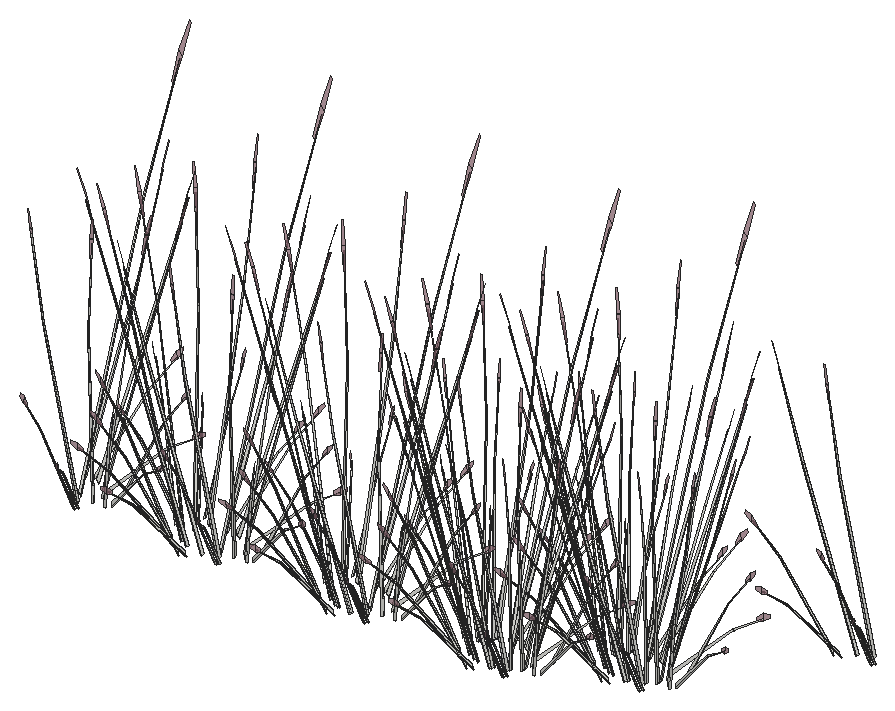
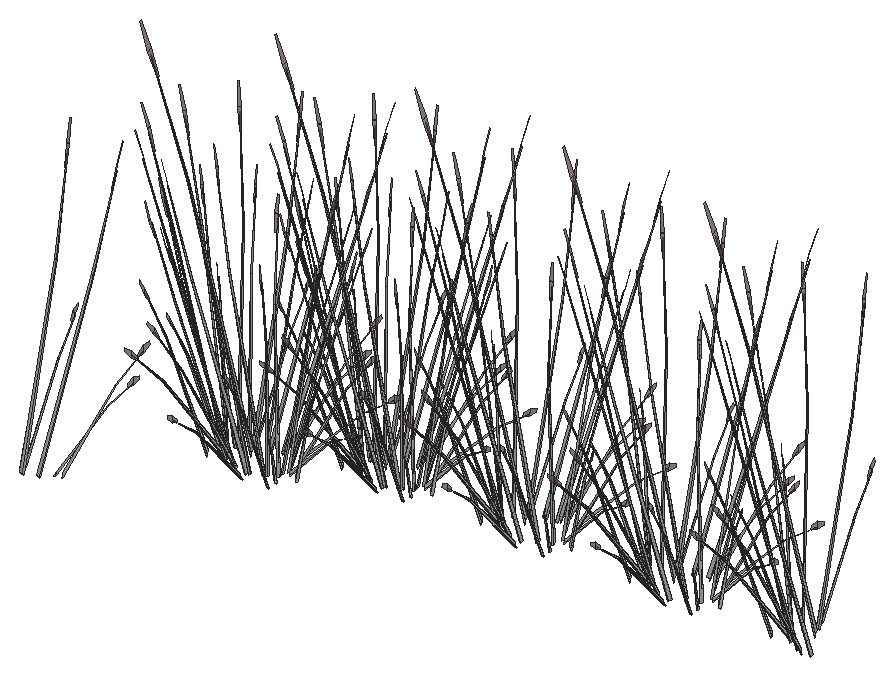
# SketchUp Ruby script. Lengths in inches.
U = 1.inch
M = Sketchup.active_model
def pt(a) = Geom::Point3d.new(a.map { |v| v * U })
def face(e, loops, mat)
  f = e.add_face(loops[0].map { |a| pt(a) })
  loops[1..].each { |l| e.add_face(l.map { |a| pt(a) }).erase! }
  f.material = f.back_material = mat if mat
  f
end
# faces: each face lists its corners as indices into pts; further lists are holes
def faces(e, pts, list, mat = nil) = list.each { |f| face(e, (f[0].is_a?(Array) ? f : [f]).map { |l| l.map { |i| pts[i] } }, mat) }
# xy, xz, yz: faces in a plane at the given z, y or x. An outline is a flat list of corners, or four numbers for a rectangle; further outlines are holes
def ring(l) = l.size == 4 ? [[l[0], l[1]], [l[2], l[1]], [l[2], l[3]], [l[0], l[3]]] : l.each_slice(2).to_a
def flat(e, list, mat, &to3) = list.each { |f| face(e, (f[0].is_a?(Array) ? f : [f]).map { |l| ring(l).map { |u, v| to3.(u, v) } }, mat) }
def xy(e, z, list, mat = nil) = flat(e, list, mat) { |x, y| [x, y, z] }
def xz(e, y, list, mat = nil) = flat(e, list, mat) { |x, z| [x, y, z] }
def yz(e, x, list, mat = nil) = flat(e, list, mat) { |y, z| [x, y, z] }
def lines(e, pts, list) = list.each { |a, b| e.add_line(pt(pts[a]), pt(pts[b])) }
# prism: a flat outline (further loops are holes) pulled along v
def prism(e, loops, v, mat = nil)
  f = face(e, loops, mat); d = Geom::Vector3d.new(v.map { |x| x * U })
  f.pushpull(f.normal.samedirection?(d) ? d.length : -d.length)
end
def box(e, o, s, mat = nil) = prism(e, [[o, [o[0] + s[0], o[1], o[2]], [o[0] + s[0], o[1] + s[1], o[2]], [o[0], o[1] + s[1], o[2]]]], [0, 0, s[2]], mat)
def at(x, y, z, deg = 0) = Geom::Transformation.translation(pt([x, y, z])) * Geom::Transformation.rotation(ORIGIN, Z_AXIS, deg.degrees)
def axes(o, x, y, z) = Geom::Transformation.new([*x, 0, *y, 0, *z, 0, *pt(o).to_a, 1])
def part(name) = M.definitions.add(name)
# library, detail: a bought-in or finely detailed component or shape, given as its bounding box
def library(name, o, s) = part(name).tap { |d| box(d.entities, o, s) }
def detail(e, o, s) = box(e.add_group.entities, o, s)
def put(e, d, t, mat = nil) = e.add_instance(d, t).tap { |i| i.material = mat if mat }
def group(e, t, mat = nil) = e.add_group.tap { |g| g.transformation = t; g.material = mat if mat }.entities
root = M.entities
M.materials.add("LightPink_Translucent").color = [144, 107, 117]
M.materials["LightPink_Translucent"].alpha = 0.75
c1 = part("blade")
p = [[2.15,0.21,22],[0,0.17,0],[0.09,0.45,0],[2.18,0.31,22],[2.29,0.31,22],[0.38,0.45,0],
  [2.48,0.24,33],[2.49,0.24,33],[2.48,0.22,33]]
faces(c1.entities,p,[[0,1,2,3],[4,5,2,3],[6,3,4,7],[8,0,3,6]])
c2 = part("seeds")
p = [[0.3,-0.1,1.38],[-0.01,-0.03,1.59],[-0.01,-0.03,0.03],[0.14,-0.07,-0.07],[0.29,-0.03,3],[0.15,0.01,3.11]]
faces(c2.entities,p,[[0,1,2,3],[1,0,4,5]],"LightPink_Translucent")
c3 = part("blade with seeds")
put(c3.entities,c1,at(0,0,0))
put(c3.entities,c2,axes([2.4,0.25,30.99],[1.5799,-0.05474,1.17369],[-0.12525,1.92788,0.29478],[-0.07173,-0.02425,1.56792]))
put(root,c3,axes([327.04,56.09,260.03],[0.74352,-0.28449,-0.1216],[0.36538,0.50492,-0.67495],[0.0981,0.21277,1.02557]))
put(root,c3,axes([330.84,50.45,259.71],[-0.07716,0.04667,1.77383],[-0.75601,-0.15746,-0.16761],[-0.02737,-0.20368,0.31391]))
put(root,c3,axes([330.24,51.8,260.03],[-0.83505,-0.03027,-0.1216],[0.02282,-0.57322,-0.67495],[0.05801,-0.22077,1.02557]))
put(root,c3,axes([329.32,52.99,259.47],[-0.65655,-0.31748,1.38283],[0.69326,-0.49431,0.59665],[0.21183,0.29789,1.33663]))
put(root,c3,axes([328.21,56.51,259.71],[0.00225,-0.07398,1.77383],[0.65113,-0.32638,-0.16761],[0.22617,0.1165,0.31391]))
put(root,c3,axes([331,50.89,259.72],[-0.00733,-0.12161,1.74944],[-0.61946,-0.35147,-0.27667],[0.09577,-0.21306,0.14031]))
put(root,c3,axes([328.81,56.07,260.03],[0.45276,-0.52302,-0.1216],[0.65568,0.30132,-0.67495],[0.22792,0.14777,1.02557]))
put(root,c3,axes([331.15,52.93,260.03],[-0.70283,-0.33692,-0.1216],[0.40491,-0.48793,-0.67495],[0.19857,-0.16961,1.02557]))
put(root,c3,axes([332.88,52.78,259.71],[-0.09924,-0.00464,1.77383],[-0.4121,-0.49725,-0.16761],[0.1655,-0.1635,0.31391]))
put(root,c3,axes([330.32,55.4,260.03],[0.04068,-0.62141,-0.1216],[0.77029,0.01698,-0.67495],[0.29667,0.04317,1.02557]))
put(root,c3,axes([331.18,54.25,260.03],[-0.38229,-0.5533,-0.1216],[0.6785,-0.2719,-0.67495],[0.28593,-0.073,1.02557]))
put(root,c3,axes([341.67,53.5625,259.72],[-0.12407,0.07933,1.74944],[0.01055,0.57963,-0.27667],[-0.2844,0.07538,0.14031]))
put(root,c3,axes([330.99,55.02,259.72],[0.16299,-0.01033,1.74944],[0.44707,-0.47471,-0.27667],[0.28992,0.06266,0.14031]))
put(root,c3,axes([340.29,54.15,259.71],[0.09697,0.01639,1.77383],[0.29997,0.53988,-0.16761],[-0.1985,0.1417,0.31391]))
put(root,c3,axes([342.25,51.15,259.71],[0.05633,0.06098,1.77383],[-0.27155,0.54815,-0.16761],[-0.27501,0.00397,0.31391]))
put(root,c3,axes([342.88,50.78,259.72],[-0.16348,-0.00431,1.74944],[-0.52047,0.43131,-0.27667],[-0.2777,-0.08813,0.14031]))
put(root,c3,axes([332.7,55.89,259.71],[-0.0687,-0.05349,1.77383],[0.15029,-0.57341,-0.16761],[0.27062,-0.03664,0.31391]))
put(root,c3,axes([342.46,53.01,260.03],[0.38229,0.5533,-0.1216],[-0.6785,0.2719,-0.67495],[-0.28593,0.073,1.02557]))
put(root,c3,axes([343.32,51.86,260.03],[-0.04068,0.62141,-0.1216],[-0.77029,-0.01698,-0.67495],[-0.29667,-0.04317,1.02557]))
put(root,c3,axes([333.26,53.38,259.72],[0.10543,-0.09307,1.74944],[-0.13495,-0.57092,-0.27667],[0.26455,-0.10825,0.14031]))
put(root,c3,axes([341.6875,55.73,259.72],[-0.01889,0.12092,1.74944],[0.53598,0.42065,-0.27667],[-0.14032,0.19892,0.14031]))
put(root,c3,axes([344.83,50.95,260.43],[-0.50709,0.58578,-0.13619],[-0.73436,-0.33748,-0.75594],[-0.25527,-0.1655,1.14864]))
put(root,c3,axes([342.49,54.33,260.03],[0.70283,0.33692,-0.1216],[-0.40491,0.48793,-0.67495],[-0.19857,0.16961,1.02557]))
put(root,c3,axes([344.63,49.56,259.71],[-0.01417,0.07324,1.77383],[-0.6991,0.2658,-0.16761],[-0.20573,-0.13587,0.31391]))
put(root,c3,axes([341.625,56.97,259.71],[0.0862,-0.03689,1.77383],[0.71245,0.24539,-0.16761],[-0.01674,0.20431,0.31391]))
put(root,c3,axes([345.43,49.84,259.72],[-0.11621,-0.08567,1.74944],[-0.77555,0.05431,-0.27667],[-0.12378,-0.20491,0.14031]))
put(root,c3,axes([343.4,55.45,260.4],[0.83505,0.03027,-0.13498],[-0.02282,0.57322,-0.74919],[-0.05801,0.22077,1.13838]))
put(root,c3,axes([346.61,51.16,260.03],[-0.74352,0.28449,-0.1216],[-0.36538,-0.50492,-0.67495],[-0.0981,-0.21277,1.02557]))
put(root,c3,axes([344.77,57.22,259.72],[0.09631,0.0984,1.74944],[0.77725,0.03866,-0.27667],[0.07816,0.217,0.14031]))
put(root,c3,axes([344.95,56.09,260.03],[0.74352,-0.28449,-0.1216],[0.36538,0.50492,-0.67495],[0.0981,0.21277,1.02557]))
put(root,c3,axes([348.74,50.45,259.71],[-0.07716,0.04667,1.77383],[-0.75601,-0.15746,-0.16761],[-0.02737,-0.20368,0.31391]))
put(root,c3,axes([348.15,51.8,260.03],[-0.83505,-0.03027,-0.1216],[0.02282,-0.57322,-0.67495],[0.05801,-0.22077,1.02557]))
put(root,c3,axes([347.23,52.99,259.47],[-0.65655,-0.31748,1.38283],[0.69326,-0.49431,0.59665],[0.21183,0.29789,1.33663]))
put(root,c3,axes([346.12,56.51,259.71],[0.00225,-0.07398,1.77383],[0.65113,-0.32638,-0.16761],[0.22617,0.1165,0.31391]))
put(root,c3,axes([348.91,50.89,259.72],[-0.00733,-0.12161,1.74944],[-0.61946,-0.35147,-0.27667],[0.09577,-0.21306,0.14031]))
put(root,c3,axes([346.71,56.07,260.03],[0.45276,-0.52302,-0.1216],[0.65568,0.30132,-0.67495],[0.22792,0.14777,1.02557]))
put(root,c3,axes([349.06,52.93,260.03],[-0.70283,-0.33692,-0.1216],[0.40491,-0.48793,-0.67495],[0.19857,-0.16961,1.02557]))
put(root,c3,axes([350.79,52.78,259.71],[-0.09924,-0.00464,1.77383],[-0.4121,-0.49725,-0.16761],[0.1655,-0.1635,0.31391]))
put(root,c3,axes([348.23,55.4,260.03],[0.04068,-0.62141,-0.1216],[0.77029,0.01698,-0.67495],[0.29667,0.04317,1.02557]))
put(root,c3,axes([349.09,54.25,260.03],[-0.38229,-0.5533,-0.1216],[0.6785,-0.2719,-0.67495],[0.28593,-0.073,1.02557]))
put(root,c3,axes([348.9,55.02,259.72],[0.16299,-0.01033,1.74944],[0.44707,-0.47471,-0.27667],[0.28992,0.06266,0.14031]))
put(root,c3,axes([360.45,53.5625,259.72],[-0.12407,0.07933,1.74944],[0.01055,0.57963,-0.27667],[-0.2844,0.07538,0.14031]))
put(root,c3,axes([350.61,55.89,259.71],[-0.0687,-0.05349,1.77383],[0.15029,-0.57341,-0.16761],[0.27062,-0.03664,0.31391]))
put(root,c3,axes([359.07,54.15,259.71],[0.09697,0.01639,1.77383],[0.29997,0.53988,-0.16761],[-0.1985,0.1417,0.31391]))
put(root,c3,axes([351.16,53.38,259.72],[0.10543,-0.09307,1.74944],[-0.13495,-0.57092,-0.27667],[0.26455,-0.10825,0.14031]))
put(root,c3,axes([361.04,51.15,259.71],[0.05633,0.06098,1.77383],[-0.27155,0.54815,-0.16761],[-0.27501,0.00397,0.31391]))
put(root,c3,axes([361.67,50.78,259.72],[-0.16348,-0.00431,1.74944],[-0.52047,0.43131,-0.27667],[-0.2777,-0.08813,0.14031]))
put(root,c3,axes([361.25,53.01,260.03],[0.38229,0.5533,-0.1216],[-0.6785,0.2719,-0.67495],[-0.28593,0.073,1.02557]))
put(root,c3,axes([362.11,51.86,260.03],[-0.04068,0.62141,-0.1216],[-0.77029,-0.01698,-0.67495],[-0.29667,-0.04317,1.02557]))
put(root,c3,axes([360.47,55.73,259.72],[-0.01889,0.12092,1.74944],[0.53598,0.42065,-0.27667],[-0.14032,0.19892,0.14031]))
put(root,c3,axes([363.61,50.95,260.43],[-0.50709,0.58578,-0.13619],[-0.73436,-0.33748,-0.75594],[-0.25527,-0.1655,1.14864]))
put(root,c3,axes([361.28,54.33,260.03],[0.70283,0.33692,-0.1216],[-0.40491,0.48793,-0.67495],[-0.19857,0.16961,1.02557]))
put(root,c3,axes([363.41,49.56,259.71],[-0.01417,0.07324,1.77383],[-0.6991,0.2658,-0.16761],[-0.20573,-0.13587,0.31391]))
put(root,c3,axes([360.41,56.97,259.71],[0.0862,-0.03689,1.77383],[0.71245,0.24539,-0.16761],[-0.01674,0.20431,0.31391]))
put(root,c3,axes([363.45,50.99,259.73],[0.34533,-0.38816,0.0643],[0.49176,0.22599,0.50621],[-0.15898,-0.12445,0.77189]))
put(root,c3,axes([364.21,49.84,259.72],[-0.11621,-0.08567,1.74944],[-0.77555,0.05431,-0.27667],[-0.12378,-0.20491,0.14031]))
put(root,c3,axes([362.18,55.45,260.4],[0.83505,0.03027,-0.13498],[-0.02282,0.57322,-0.74919],[-0.05801,0.22077,1.13838]))
put(root,c3,axes([365.39,51.16,260.03],[-0.74352,0.28449,-0.1216],[-0.36538,-0.50492,-0.67495],[-0.0981,-0.21277,1.02557]))
put(root,c3,axes([363.55,57.22,259.72],[0.09631,0.0984,1.74944],[0.77725,0.03866,-0.27667],[0.07816,0.217,0.14031]))
put(root,c3,axes([363.73,56.09,260.03],[0.74352,-0.28449,-0.1216],[0.36538,0.50492,-0.67495],[0.0981,0.21277,1.02557]))
put(root,c3,axes([367.53,50.45,259.71],[-0.07716,0.04667,1.77383],[-0.75601,-0.15746,-0.16761],[-0.02737,-0.20368,0.31391]))
put(root,c3,axes([366.93,51.8,260.03],[-0.83505,-0.03027,-0.1216],[0.02282,-0.57322,-0.67495],[0.05801,-0.22077,1.02557]))
put(root,c3,axes([366.01,52.99,259.47],[-0.65655,-0.31748,1.38283],[0.69326,-0.49431,0.59665],[0.21183,0.29789,1.33663]))
put(root,c3,axes([364.9,56.51,259.71],[0.00225,-0.07398,1.77383],[0.65113,-0.32638,-0.16761],[0.22617,0.1165,0.31391]))
put(root,c3,axes([367.69,50.89,259.72],[-0.00733,-0.12161,1.74944],[-0.61946,-0.35147,-0.27667],[0.09577,-0.21306,0.14031]))
put(root,c3,axes([365.5,56.07,260.03],[0.45276,-0.52302,-0.1216],[0.65568,0.30132,-0.67495],[0.22792,0.14777,1.02557]))
put(root,c3,axes([367.84,52.93,260.03],[-0.70283,-0.33692,-0.1216],[0.40491,-0.48793,-0.67495],[0.19857,-0.16961,1.02557]))
put(root,c3,axes([369.57,52.78,259.71],[-0.09924,-0.00464,1.77383],[-0.4121,-0.49725,-0.16761],[0.1655,-0.1635,0.31391]))
put(root,c3,axes([367.01,55.4,260.03],[0.04068,-0.62141,-0.1216],[0.77029,0.01698,-0.67495],[0.29667,0.04317,1.02557]))
put(root,c3,axes([367.87,54.25,260.03],[-0.38229,-0.5533,-0.1216],[0.6785,-0.2719,-0.67495],[0.28593,-0.073,1.02557]))
put(root,c3,axes([378.09,53.5625,259.72],[-0.12407,0.07933,1.74944],[0.01055,0.57963,-0.27667],[-0.2844,0.07538,0.14031]))
put(root,c3,axes([367.68,55.02,259.72],[0.16299,-0.01033,1.74944],[0.44707,-0.47471,-0.27667],[0.28992,0.06266,0.14031]))
put(root,c3,axes([376.71,54.15,259.71],[0.09697,0.01639,1.77383],[0.29997,0.53988,-0.16761],[-0.1985,0.1417,0.31391]))
put(root,c3,axes([378.67,51.15,259.71],[0.05633,0.06098,1.77383],[-0.27155,0.54815,-0.16761],[-0.27501,0.00397,0.31391]))
put(root,c3,axes([379.3,50.78,259.72],[-0.16348,-0.00431,1.74944],[-0.52047,0.43131,-0.27667],[-0.2777,-0.08813,0.14031]))
put(root,c3,axes([378.88,53.01,260.03],[0.38229,0.5533,-0.1216],[-0.6785,0.2719,-0.67495],[-0.28593,0.073,1.02557]))
put(root,c3,axes([379.74,51.86,260.03],[-0.04068,0.62141,-0.1216],[-0.77029,-0.01698,-0.67495],[-0.29667,-0.04317,1.02557]))
put(root,c3,axes([378.58,53.02,259.73],[-0.27906,-0.41663,0.0643],[0.50888,-0.20393,0.50621],[-0.22432,0.04024,0.77189]))
put(root,c3,axes([369.39,55.89,259.71],[-0.0687,-0.05349,1.77383],[0.15029,-0.57341,-0.16761],[0.27062,-0.03664,0.31391]))
put(root,c3,axes([369.95,53.38,259.72],[0.10543,-0.09307,1.74944],[-0.13495,-0.57092,-0.27667],[0.26455,-0.10825,0.14031]))
put(root,c3,axes([378.65,54.45,259.73],[-0.52161,-0.25698,0.0643],[0.30368,-0.36595,0.50621],[-0.16723,0.11831,0.77189]))
put(root,c3,axes([379.47,51.76,259.73],[0.03826,-0.46465,0.0643],[0.57772,0.01274,0.50621],[-0.2213,-0.04862,0.77189]))
put(root,c3,axes([378.11,55.73,259.72],[-0.01889,0.12092,1.74944],[0.53598,0.42065,-0.27667],[-0.14032,0.19892,0.14031]))
put(root,c3,axes([381.25,50.95,260.43],[-0.50709,0.58578,-0.13619],[-0.73436,-0.33748,-0.75594],[-0.25527,-0.1655,1.14864]))
put(root,c3,axes([378.91,54.33,260.03],[0.70283,0.33692,-0.1216],[-0.40491,0.48793,-0.67495],[-0.19857,0.16961,1.02557]))
put(root,c3,axes([381.05,49.56,259.71],[-0.01417,0.07324,1.77383],[-0.6991,0.2658,-0.16761],[-0.20573,-0.13587,0.31391]))
put(root,c3,axes([379.68,55.66,259.73],[-0.62439,-0.02847,0.0643],[0.01712,-0.42991,0.50621],[-0.06534,0.16468,0.77189]))
put(root,c3,axes([378.05,56.97,259.71],[0.0862,-0.03689,1.77383],[0.71245,0.24539,-0.16761],[-0.01674,0.20431,0.31391]))
put(root,c3,axes([381.09,50.99,259.73],[0.34533,-0.38816,0.0643],[0.49176,0.22599,0.50621],[-0.15898,-0.12445,0.77189]))
put(root,c3,axes([381.84,49.84,259.72],[-0.11621,-0.08567,1.74944],[-0.77555,0.05431,-0.27667],[-0.12378,-0.20491,0.14031]))
put(root,c3,axes([379.82,55.45,260.4],[0.83505,0.03027,-0.13498],[-0.02282,0.57322,-0.74919],[-0.05801,0.22077,1.13838]))
put(root,c3,axes([383.02,51.16,260.03],[-0.74352,0.28449,-0.1216],[-0.36538,-0.50492,-0.67495],[-0.0981,-0.21277,1.02557]))
put(root,c3,axes([381.38,56.32,259.73],[-0.55987,0.20767,0.0643],[-0.27403,-0.37869,0.50621],[0.05407,0.16693,0.77189]))
put(root,c3,axes([383.01,50.94,259.73],[0.55987,-0.20767,0.0643],[0.27403,0.37869,0.50621],[-0.05407,-0.16693,0.77189]))
put(root,c3,axes([381.1875,57.22,259.72],[0.09631,0.0984,1.74944],[0.77725,0.03866,-0.27667],[0.07816,0.217,0.14031]))
put(root,c3,axes([381.36,56.09,260.03],[0.74352,-0.28449,-0.1216],[0.36538,0.50492,-0.67495],[0.0981,0.21277,1.02557]))
put(root,c3,axes([385.16,50.45,259.71],[-0.07716,0.04667,1.77383],[-0.75601,-0.15746,-0.16761],[-0.02737,-0.20368,0.31391]))
put(root,c3,axes([384.57,51.8,260.03],[-0.83505,-0.03027,-0.1216],[0.02282,-0.57322,-0.67495],[0.05801,-0.22077,1.02557]))
put(root,c3,axes([390.22,59.79,259.72],[-0.12407,0.07933,1.74944],[0.01055,0.57963,-0.27667],[-0.2844,0.07538,0.14031]))
put(root,c3,axes([388.84,60.375,259.71],[0.09697,0.01639,1.77383],[0.29997,0.53988,-0.16761],[-0.1985,0.1417,0.31391]))
put(root,c3,axes([383.3,56.26,259.73],[-0.34533,0.38816,0.0643],[-0.49176,-0.22599,0.50621],[0.15898,0.12445,0.77189]))
put(root,c3,axes([390.8,57.38,259.71],[0.05633,0.06098,1.77383],[-0.27155,0.54815,-0.16761],[-0.27501,0.00397,0.31391]))
put(root,c3,axes([391.43,57.01,259.72],[-0.16348,-0.00431,1.74944],[-0.52047,0.43131,-0.27667],[-0.2777,-0.08813,0.14031]))
put(root,c3,axes([391.01,59.24,260.03],[0.38229,0.5533,-0.1216],[-0.6785,0.2719,-0.67495],[-0.28593,0.073,1.02557]))
put(root,c3,axes([391.87,58.09,260.03],[-0.04068,0.62141,-0.1216],[-0.77029,-0.01698,-0.67495],[-0.29667,-0.04317,1.02557]))
put(root,c3,axes([390.71,59.25,259.73],[-0.27906,-0.41663,0.0643],[0.50888,-0.20393,0.50621],[-0.22432,0.04024,0.77189]))
put(root,c3,axes([383.64,52.99,259.47],[-0.65655,-0.31748,1.38283],[0.69326,-0.49431,0.59665],[0.21183,0.29789,1.33663]))
put(root,c3,axes([382.54,56.51,259.71],[0.00225,-0.07398,1.77383],[0.65113,-0.32638,-0.16761],[0.22617,0.1165,0.31391]))
put(root,c3,axes([384.71,51.6,259.73],[0.62439,0.02847,0.0643],[-0.01712,0.42991,0.50621],[0.06534,-0.16468,0.77189]))
put(root,c3,axes([385.33,50.89,259.72],[-0.00733,-0.12161,1.74944],[-0.61946,-0.35147,-0.27667],[0.09577,-0.21306,0.14031]))
put(root,c3,axes([390.79,60.68,259.73],[-0.52161,-0.25698,0.0643],[0.30368,-0.36595,0.50621],[-0.16723,0.11831,0.77189]))
put(root,c3,axes([391.6,57.98,259.73],[0.03826,-0.46465,0.0643],[0.57772,0.01274,0.50621],[-0.2213,-0.04862,0.77189]))
put(root,c3,axes([390.24,61.95,259.72],[-0.01889,0.12092,1.74944],[0.53598,0.42065,-0.27667],[-0.14032,0.19892,0.14031]))
put(root,c3,axes([393.375,57.18,260.43],[-0.50709,0.58578,-0.13619],[-0.73436,-0.33748,-0.75594],[-0.25527,-0.1655,1.14864]))
put(root,c3,axes([383.13,56.07,260.03],[0.45276,-0.52302,-0.1216],[0.65568,0.30132,-0.67495],[0.22792,0.14777,1.02557]))
put(root,c3,axes([385.48,52.93,260.03],[-0.70283,-0.33692,-0.1216],[0.40491,-0.48793,-0.67495],[0.19857,-0.16961,1.02557]))
put(root,c3,axes([391.04,60.55,260.03],[0.70283,0.33692,-0.1216],[-0.40491,0.48793,-0.67495],[-0.19857,0.16961,1.02557]))
put(root,c3,axes([384.92,55.5,259.73],[-0.03826,0.46465,0.0643],[-0.57772,-0.01274,0.50621],[0.2213,0.04862,0.77189]))
put(root,c3,axes([393.18,55.79,259.71],[-0.01417,0.07324,1.77383],[-0.6991,0.2658,-0.16761],[-0.20573,-0.13587,0.31391]))
put(root,c3,axes([385.73,52.81,259.73],[0.52161,0.25698,0.0643],[-0.30368,0.36595,0.50621],[0.16723,-0.11831,0.77189]))
put(root,c3,axes([391.8125,61.88,259.73],[-0.62439,-0.02847,0.0643],[0.01712,-0.42991,0.50621],[-0.06534,0.16468,0.77189]))
put(root,c3,axes([387.21,52.78,259.71],[-0.09924,-0.00464,1.77383],[-0.4121,-0.49725,-0.16761],[0.1655,-0.1635,0.31391]))
put(root,c3,axes([390.18,63.19,259.71],[0.0862,-0.03689,1.77383],[0.71245,0.24539,-0.16761],[-0.01674,0.20431,0.31391]))
put(root,c3,axes([385.8125,54.23,259.73],[0.27906,0.41663,0.0643],[-0.50888,0.20393,0.50621],[0.22432,-0.04024,0.77189]))
put(root,c3,axes([384.65,55.4,260.03],[0.04068,-0.62141,-0.1216],[0.77029,0.01698,-0.67495],[0.29667,0.04317,1.02557]))
put(root,c3,axes([385.51,54.25,260.03],[-0.38229,-0.5533,-0.1216],[0.6785,-0.2719,-0.67495],[0.28593,-0.073,1.02557]))
put(root,c3,axes([385.32,55.02,259.72],[0.16299,-0.01033,1.74944],[0.44707,-0.47471,-0.27667],[0.28992,0.06266,0.14031]))
put(root,c3,axes([393.22,57.22,259.73],[0.34533,-0.38816,0.0643],[0.49176,0.22599,0.50621],[-0.15898,-0.12445,0.77189]))
put(root,c3,axes([393.98,56.07,259.72],[-0.11621,-0.08567,1.74944],[-0.77555,0.05431,-0.27667],[-0.12378,-0.20491,0.14031]))
put(root,c3,axes([387.03,55.89,259.71],[-0.0687,-0.05349,1.77383],[0.15029,-0.57341,-0.16761],[0.27062,-0.03664,0.31391]))
put(root,c3,axes([391.95,61.68,260.4],[0.83505,0.03027,-0.13498],[-0.02282,0.57322,-0.74919],[-0.05801,0.22077,1.13838]))
put(root,c3,axes([395.16,57.39,260.03],[-0.74352,0.28449,-0.1216],[-0.36538,-0.50492,-0.67495],[-0.0981,-0.21277,1.02557]))
put(root,c3,axes([387.58,53.38,259.72],[0.10543,-0.09307,1.74944],[-0.13495,-0.57092,-0.27667],[0.26455,-0.10825,0.14031]))
put(root,c3,axes([393.51,62.55,259.73],[-0.55987,0.20767,0.0643],[-0.27403,-0.37869,0.50621],[0.05407,0.16693,0.77189]))
put(root,c3,axes([395.14,57.16,259.73],[0.55987,-0.20767,0.0643],[0.27403,0.37869,0.50621],[-0.05407,-0.16693,0.77189]))
put(root,c3,axes([393.32,63.45,259.72],[0.09631,0.0984,1.74944],[0.77725,0.03866,-0.27667],[0.07816,0.217,0.14031]))
put(root,c3,axes([393.5,62.32,260.03],[0.74352,-0.28449,-0.1216],[0.36538,0.50492,-0.67495],[0.0981,0.21277,1.02557]))
put(root,c3,axes([397.29,56.68,259.71],[-0.07716,0.04667,1.77383],[-0.75601,-0.15746,-0.16761],[-0.02737,-0.20368,0.31391]))
put(root,c3,axes([396.7,58.03,260.03],[-0.83505,-0.03027,-0.1216],[0.02282,-0.57322,-0.67495],[0.05801,-0.22077,1.02557]))
put(root,c3,axes([395.43,62.49,259.73],[-0.34533,0.38816,0.0643],[-0.49176,-0.22599,0.50621],[0.15898,0.12445,0.77189]))
put(root,c3,axes([395.77,59.21,259.47],[-0.65655,-0.31748,1.38283],[0.69326,-0.49431,0.59665],[0.21183,0.29789,1.33663]))
put(root,c3,axes([394.67,62.73,259.71],[0.00225,-0.07398,1.77383],[0.65113,-0.32638,-0.16761],[0.22617,0.1165,0.31391]))
put(root,c3,axes([396.84,57.83,259.73],[0.62439,0.02847,0.0643],[-0.01712,0.42991,0.50621],[0.06534,-0.16468,0.77189]))
put(root,c3,axes([397.46,57.12,259.72],[-0.00733,-0.12161,1.74944],[-0.61946,-0.35147,-0.27667],[0.09577,-0.21306,0.14031]))
put(root,c3,axes([395.26,62.3,260.03],[0.45276,-0.52302,-0.1216],[0.65568,0.30132,-0.67495],[0.22792,0.14777,1.02557]))
put(root,c3,axes([397.61,59.16,260.03],[-0.70283,-0.33692,-0.1216],[0.40491,-0.48793,-0.67495],[0.19857,-0.16961,1.02557]))
put(root,c3,axes([397.05,61.73,259.73],[-0.03826,0.46465,0.0643],[-0.57772,-0.01274,0.50621],[0.2213,0.04862,0.77189]))
put(root,c3,axes([397.87,59.03,259.73],[0.52161,0.25698,0.0643],[-0.30368,0.36595,0.50621],[0.16723,-0.11831,0.77189]))
put(root,c3,axes([399.34,59.01,259.71],[-0.09924,-0.00464,1.77383],[-0.4121,-0.49725,-0.16761],[0.1655,-0.1635,0.31391]))
put(root,c3,axes([397.94,60.46,259.73],[0.27906,0.41663,0.0643],[-0.50888,0.20393,0.50621],[0.22432,-0.04024,0.77189]))
put(root,c3,axes([396.78,61.62,260.03],[0.04068,-0.62141,-0.1216],[0.77029,0.01698,-0.67495],[0.29667,0.04317,1.02557]))
put(root,c3,axes([397.64,60.47,260.03],[-0.38229,-0.5533,-0.1216],[0.6785,-0.2719,-0.67495],[0.28593,-0.073,1.02557]))
put(root,c3,axes([397.45,61.25,259.72],[0.16299,-0.01033,1.74944],[0.44707,-0.47471,-0.27667],[0.28992,0.06266,0.14031]))
put(root,c3,axes([407.8,74.22,259.71],[-0.01417,0.07324,1.77383],[-0.6991,0.2658,-0.16761],[-0.20573,-0.13587,0.31391]))
put(root,c3,axes([399.16,62.12,259.71],[-0.0687,-0.05349,1.77383],[0.15029,-0.57341,-0.16761],[0.27062,-0.03664,0.31391]))
put(root,c3,axes([399.71,59.61,259.72],[0.10543,-0.09307,1.74944],[-0.13495,-0.57092,-0.27667],[0.26455,-0.10825,0.14031]))
put(root,c3,axes([408.59,74.5,259.72],[-0.11621,-0.08567,1.74944],[-0.77555,0.05431,-0.27667],[-0.12378,-0.20491,0.14031]))
put(root,c3,axes([409.77,75.82,260.03],[-0.74352,0.28449,-0.1216],[-0.36538,-0.50492,-0.67495],[-0.0981,-0.21277,1.02557]))
put(root,c3,axes([411.91,75.12,259.71],[-0.07716,0.04667,1.77383],[-0.75601,-0.15746,-0.16761],[-0.02737,-0.20368,0.31391]))
put(root,c3,axes([411.32,76.46,260.03],[-0.83505,-0.03027,-0.1216],[0.02282,-0.57322,-0.67495],[0.05801,-0.22077,1.02557]))
put(root,c3,axes([412.08,75.55,259.72],[-0.00733,-0.12161,1.74944],[-0.61946,-0.35147,-0.27667],[0.09577,-0.21306,0.14031]))
